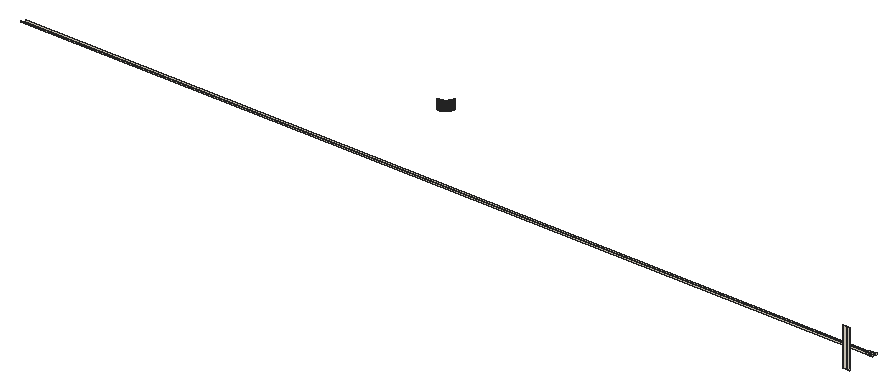
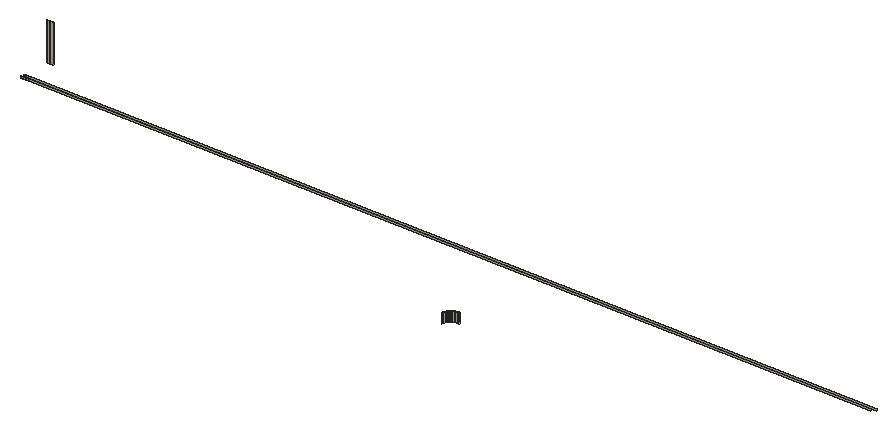
# SketchUp Ruby script. Lengths in inches.
U = 1.inch
M = Sketchup.active_model
def pt(a) = Geom::Point3d.new(a.map { |v| v * U })
def face(e, loops, mat)
  f = e.add_face(loops[0].map { |a| pt(a) })
  loops[1..].each { |l| e.add_face(l.map { |a| pt(a) }).erase! }
  f.material = f.back_material = mat if mat
  f
end
# faces: each face lists its corners as indices into pts; further lists are holes
def faces(e, pts, list, mat = nil) = list.each { |f| face(e, (f[0].is_a?(Array) ? f : [f]).map { |l| l.map { |i| pts[i] } }, mat) }
# xy, xz, yz: faces in a plane at the given z, y or x. An outline is a flat list of corners, or four numbers for a rectangle; further outlines are holes
def ring(l) = l.size == 4 ? [[l[0], l[1]], [l[2], l[1]], [l[2], l[3]], [l[0], l[3]]] : l.each_slice(2).to_a
def flat(e, list, mat, &to3) = list.each { |f| face(e, (f[0].is_a?(Array) ? f : [f]).map { |l| ring(l).map { |u, v| to3.(u, v) } }, mat) }
def xy(e, z, list, mat = nil) = flat(e, list, mat) { |x, y| [x, y, z] }
def xz(e, y, list, mat = nil) = flat(e, list, mat) { |x, z| [x, y, z] }
def yz(e, x, list, mat = nil) = flat(e, list, mat) { |y, z| [x, y, z] }
def lines(e, pts, list) = list.each { |a, b| e.add_line(pt(pts[a]), pt(pts[b])) }
# prism: a flat outline (further loops are holes) pulled along v
def prism(e, loops, v, mat = nil)
  f = face(e, loops, mat); d = Geom::Vector3d.new(v.map { |x| x * U })
  f.pushpull(f.normal.samedirection?(d) ? d.length : -d.length)
end
def box(e, o, s, mat = nil) = prism(e, [[o, [o[0] + s[0], o[1], o[2]], [o[0] + s[0], o[1] + s[1], o[2]], [o[0], o[1] + s[1], o[2]]]], [0, 0, s[2]], mat)
def at(x, y, z, deg = 0) = Geom::Transformation.translation(pt([x, y, z])) * Geom::Transformation.rotation(ORIGIN, Z_AXIS, deg.degrees)
def axes(o, x, y, z) = Geom::Transformation.new([*x, 0, *y, 0, *z, 0, *pt(o).to_a, 1])
def part(name) = M.definitions.add(name)
# library, detail: a bought-in or finely detailed component or shape, given as its bounding box
def library(name, o, s) = part(name).tap { |d| box(d.entities, o, s) }
def detail(e, o, s) = box(e.add_group.entities, o, s)
def put(e, d, t, mat = nil) = e.add_instance(d, t).tap { |i| i.material = mat if mat }
def group(e, t, mat = nil) = e.add_group.tap { |g| g.transformation = t; g.material = mat if mat }.entities
root = M.entities
M.materials.add("0027 AP L140 CRUSHED ICE").color = [241, 233, 217]
xz(root,216,[[345,120,345.375,132]],"0027 AP L140 CRUSHED ICE")
xz(root,225,[[78,120,345,120.5],[345,120,345.28,120.5]],"0027 AP L140 CRUSHED ICE")
xz(root,225.01,[[345.57,120,345.85,120.5]],"0027 AP L140 CRUSHED ICE")
xz(root,226,[[79,120,345,120.5],[345,120,345.27,120.5]],"0027 AP L140 CRUSHED ICE")
xz(root,226.01,[[345.54,120,345.82,120.5]],"0027 AP L140 CRUSHED ICE")
xz(root,255,[[185.84,120,185.92,123],[185.92,120,186,123],[186,120,186.08,123],[186.08,120,186.16,123]],"0027 AP L140 CRUSHED ICE")
p = [[345.75,216.01,132],[345.375,216,132],[345.375,216,120],[345.75,216.01,120],[346.13,216.02,132],[346.13,216.02,120],
  [346.51,216.03,132],[346.51,216.03,120],[346.88,216.05,132],[346.88,216.05,120],[347.26,216.07,132],[347.26,216.07,120],
  [345.57,225.01,120],[345.28,225,120],[345.28,225,120.5],[345.57,225.01,120.5],[346.13,225.02,120],[345.85,225.01,120],
  [345.85,225.01,120.5],[346.13,225.02,120.5],[346.41,225.04,120],[346.41,225.04,120.5],[346.7,225.05,120],[346.7,225.05,120.5],
  [346.98,225.07,120],[346.98,225.07,120.5],[347.26,225.09,120],[347.26,225.09,120.5],[345.27,226,120],[345.54,226.01,120],
  [345.54,226.01,120.5],[345.27,226,120.5],[345.82,226.01,120],[346.09,226.02,120],[346.09,226.02,120.5],[345.82,226.01,120.5],
  [346.36,226.04,120],[346.36,226.04,120.5],[346.63,226.05,120],[346.63,226.05,120.5],[346.9,226.07,120],[346.9,226.07,120.5],
  [347.18,226.09,120],[347.18,226.09,120.5],[347.45,226.12,120],[347.45,226.12,120.5],[185.6875,255.02,120],[185.61,255.03,120],
  [185.61,255.03,123],[185.6875,255.02,123],[185.76,255.01,120],[185.76,255.01,123],[185.84,255,120],[185.84,255,123],
  [186.24,255.01,120],[186.16,255,120],[186.16,255,123],[186.24,255.01,123],[186.3125,255.02,120],[186.3125,255.02,123],
  [186.39,255.03,120],[186.39,255.03,123],[186.47,255.04,120],[186.47,255.04,123],[186.55,255.05,120],[186.55,255.05,123],
  [186.625,255.07,120],[186.625,255.07,123],[186.7,255.08,120],[186.7,255.08,123],[186.78,255.1,120],[186.78,255.1,123],
  [186.85,255.125,120],[186.85,255.125,123],[186.93,255.15,120],[186.93,255.15,123],[187,255.17,120],[187,255.17,123],
  [187.08,255.2,120],[187.08,255.2,123],[187.15,255.23,120],[187.15,255.23,123],[187.22,255.26,120],[187.22,255.26,123],
  [187.29,255.29,120],[187.29,255.29,123],[187.36,255.33,120],[187.36,255.33,123],[187.43,255.36,120],[187.43,255.36,123],
  [187.5,255.4,120],[187.5,255.4,123],[187.57,255.44,120],[187.57,255.44,123],[187.63,255.48,120],[187.63,255.48,123],
  [187.7,255.53,120],[187.7,255.53,123],[187.76,255.57,120],[187.76,255.57,123],[187.83,255.62,120],[187.83,255.62,123],
  [187.89,255.67,120],[187.89,255.67,123],[187.95,255.72,120],[187.95,255.72,123],[188.01,255.77,120],[188.01,255.77,123],
  [188.07,255.82,120],[188.07,255.82,123],[188.12,255.88,120],[188.12,255.88,123],[188.18,255.93,120],[188.18,255.93,123],
  [188.23,255.99,120],[188.23,255.99,123],[188.28,256.05,120],[188.28,256.05,123],[188.33,256.11,120],[188.33,256.11,123],
  [188.38,256.17,120],[188.38,256.17,123],[188.43,256.24,120],[188.43,256.24,123],[188.47,256.3,120],[188.47,256.3,123],
  [188.52,256.37,120],[188.52,256.37,123],[188.56,256.43,120],[188.56,256.43,123],[188.6,256.5,120],[188.6,256.5,123],
  [188.64,256.57,120],[188.64,256.57,123],[188.67,256.64,120],[188.67,256.64,123],[188.71,256.71,120],[188.71,256.71,123],
  [188.74,256.78,120],[188.74,256.78,123],[188.77,256.85,120],[188.77,256.85,123],[188.8,256.92,120],[188.8,256.92,123],
  [188.83,257,120],[188.83,257,123],[188.85,257.07,120],[188.85,257.07,123],[188.875,257.15,120],[188.875,257.15,123],
  [188.9,257.22,120],[188.9,257.22,123],[188.92,257.3,120],[188.92,257.3,123],[188.93,257.375,120],[188.93,257.375,123],
  [188.95,257.45,120],[188.95,257.45,123],[188.96,257.53,120],[188.96,257.53,123],[188.97,257.61,120],[188.97,257.61,123],
  [188.98,257.6875,120],[188.98,257.6875,123]]
faces(root,p,[[0,1,2,3],[4,0,3,5],[6,4,5,7],[8,6,7,9],[10,8,9,11],[12,13,14,15],[16,17,18,19],[20,16,19,21],
  [22,20,21,23],[24,22,23,25],[26,24,25,27],[28,29,30,31],[32,33,34,35],[33,36,37,34],[36,38,39,37],[38,40,41,39],
  [40,42,43,41],[42,44,45,43],[46,47,48,49],[50,46,49,51],[52,50,51,53],[54,55,56,57],[58,54,57,59],[60,58,59,61],
  [62,60,61,63],[64,62,63,65],[66,64,65,67],[68,66,67,69],[70,68,69,71],[72,70,71,73],[74,72,73,75],[76,74,75,77],
  [78,76,77,79],[80,78,79,81],[82,80,81,83],[84,82,83,85],[86,84,85,87],[88,86,87,89],[90,88,89,91],[92,90,91,93],
  [94,92,93,95],[96,94,95,97],[98,96,97,99],[100,98,99,101],[102,100,101,103],[104,102,103,105],[106,104,105,107],[108,106,107,109],
  [110,108,109,111],[112,110,111,113],[114,112,113,115],[116,114,115,117],[118,116,117,119],[120,118,119,121],[122,120,121,123],[124,122,123,125],
  [126,124,125,127],[128,126,127,129],[130,128,129,131],[132,130,131,133],[134,132,133,135],[136,134,135,137],[138,136,137,139],[140,138,139,141],
  [142,140,141,143],[144,142,143,145],[146,144,145,147],[148,146,147,149],[150,148,149,151],[152,150,151,153],[154,152,153,155],[156,154,155,157],
  [158,156,157,159],[160,158,159,161],[162,160,161,163]],"0027 AP L140 CRUSHED ICE")
